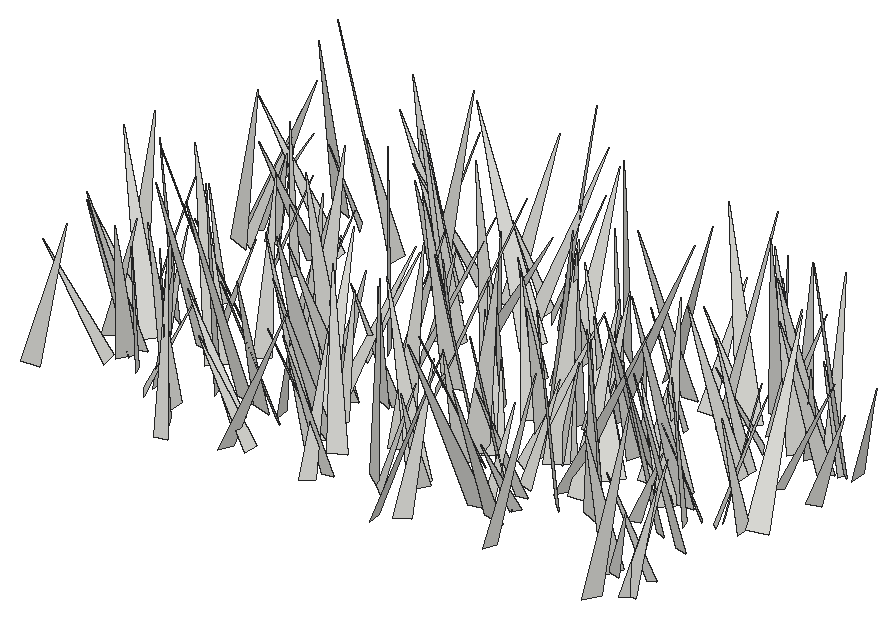
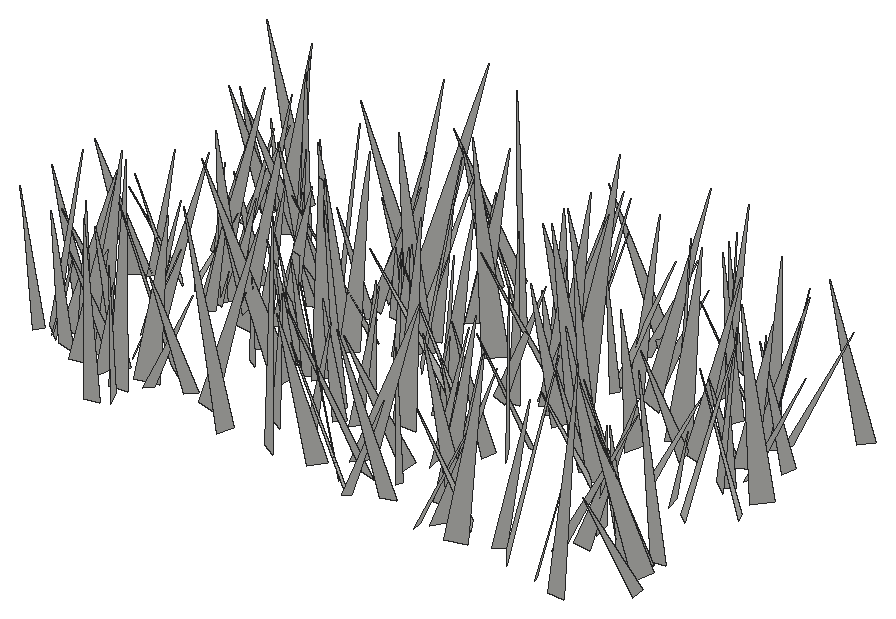
# SketchUp Ruby script. Lengths in inches.
U = 1.inch
M = Sketchup.active_model
def pt(a) = Geom::Point3d.new(a.map { |v| v * U })
def face(e, loops, mat)
  f = e.add_face(loops[0].map { |a| pt(a) })
  loops[1..].each { |l| e.add_face(l.map { |a| pt(a) }).erase! }
  f.material = f.back_material = mat if mat
  f
end
# faces: each face lists its corners as indices into pts; further lists are holes
def faces(e, pts, list, mat = nil) = list.each { |f| face(e, (f[0].is_a?(Array) ? f : [f]).map { |l| l.map { |i| pts[i] } }, mat) }
# xy, xz, yz: faces in a plane at the given z, y or x. An outline is a flat list of corners, or four numbers for a rectangle; further outlines are holes
def ring(l) = l.size == 4 ? [[l[0], l[1]], [l[2], l[1]], [l[2], l[3]], [l[0], l[3]]] : l.each_slice(2).to_a
def flat(e, list, mat, &to3) = list.each { |f| face(e, (f[0].is_a?(Array) ? f : [f]).map { |l| ring(l).map { |u, v| to3.(u, v) } }, mat) }
def xy(e, z, list, mat = nil) = flat(e, list, mat) { |x, y| [x, y, z] }
def xz(e, y, list, mat = nil) = flat(e, list, mat) { |x, z| [x, y, z] }
def yz(e, x, list, mat = nil) = flat(e, list, mat) { |y, z| [x, y, z] }
def lines(e, pts, list) = list.each { |a, b| e.add_line(pt(pts[a]), pt(pts[b])) }
# prism: a flat outline (further loops are holes) pulled along v
def prism(e, loops, v, mat = nil)
  f = face(e, loops, mat); d = Geom::Vector3d.new(v.map { |x| x * U })
  f.pushpull(f.normal.samedirection?(d) ? d.length : -d.length)
end
def box(e, o, s, mat = nil) = prism(e, [[o, [o[0] + s[0], o[1], o[2]], [o[0] + s[0], o[1] + s[1], o[2]], [o[0], o[1] + s[1], o[2]]]], [0, 0, s[2]], mat)
def at(x, y, z, deg = 0) = Geom::Transformation.translation(pt([x, y, z])) * Geom::Transformation.rotation(ORIGIN, Z_AXIS, deg.degrees)
def axes(o, x, y, z) = Geom::Transformation.new([*x, 0, *y, 0, *z, 0, *pt(o).to_a, 1])
def part(name) = M.definitions.add(name)
# library, detail: a bought-in or finely detailed component or shape, given as its bounding box
def library(name, o, s) = part(name).tap { |d| box(d.entities, o, s) }
def detail(e, o, s) = box(e.add_group.entities, o, s)
def put(e, d, t, mat = nil) = e.add_instance(d, t).tap { |i| i.material = mat if mat }
def group(e, t, mat = nil) = e.add_group.tap { |g| g.transformation = t; g.material = mat if mat }.entities
root = M.entities
c1 = part("fur_instance\#9")
p = [[0.8125,0,1.79],[0.67,-0.02,1.48],[0,-0.11,0],[0,0.11,0]]
faces(c1.entities,p,[[0,1,2,3]])
put(root,c1,axes([510.49,407.03,-21.66],[0.64289,6.12986,1.03372],[6.0316,-0.86662,1.38779],[-1.50455,-0.85491,6.00521]))
put(root,c1,axes([545.08,408,-21.66],[6.61649,-1.70465,2.3436],[-2.13195,-6.81989,1.0584],[-1.96294,1.66119,6.75008]))
put(root,c1,axes([515.89,409.48,-21.66],[-4.18794,0.93567,0.33129],[0.9893,4.05153,1.06324],[0.08071,-1.11073,4.15738]))
put(root,c1,axes([514.51,408.66,-21.66],[6.16079,-1.33707,0.34037],[-1.37023,-6.11166,0.79308],[-0.16154,0.84778,6.25413]))
put(root,c1,axes([527.73,407.37,-21.66],[6.18202,1.83786,0.77531],[1.68935,-6.16651,1.14736],[-1.06062,0.8903,6.34654]))
put(root,c1,axes([521.85,409.94,-21.66],[-1.08629,-5.09453,1.21583],[-5.17343,0.84989,-1.06105],[-0.81738,1.39139,5.09985]))
put(root,c1,axes([533.82,412.02,-21.66],[-0.13701,-6.93499,0.01519],[-6.899,0.13785,0.70555],[0.70571,0.00117,6.90036]))
put(root,c1,axes([509.59,409.04,-21.66],[4.32475,3.25099,2.86901],[3.37923,-5.06616,0.64681],[-2.71679,-1.12634,5.37159]))
put(root,c1,axes([532.06,412.72,-21.66],[1.01288,-8.11783,0.06805],[-8.08119,-1.01477,-0.77093],[-0.77341,-0.02823,8.14437]))
put(root,c1,axes([497.83,409.4,-21.66],[-1.7832,4.7887,2.83203],[5.02838,2.65983,-1.33139],[2.38064,-2.03113,4.93345]))
put(root,c1,axes([529.11,408.52,-21.66],[4.10356,-2.98524,2.70877],[-3.77942,-4.1935,1.10399],[-1.40181,2.56732,4.95298]))
put(root,c1,axes([544.13,411.4,-21.66],[4.71186,-4.25626,1.34995],[-4.06485,-4.9009,-1.26409],[-1.848,-0.07223,6.22249]))
put(root,c1,axes([546.75,409.71,-21.66],[-0.57371,3.97778,1.97621],[4.19128,1.14438,-1.08668],[1.47014,-1.71025,3.86924]))
put(root,c1,axes([508.65,410.58,-21.66],[-6.63003,0.58928,2.6026],[0.94805,7.03587,0.82207],[2.49439,-1.10786,6.6052]))
put(root,c1,axes([521.1875,408.62,-21.66],[-4.05743,3.11883,1.27429],[2.94276,4.25195,-1.03673],[1.64046,0.08657,5.0115]))
put(root,c1,axes([544.29,411.24,-21.66],[0.84418,-3.62493,0.18375],[-3.45271,-0.74384,1.18829],[1.11924,0.43944,3.52714]))
put(root,c1,axes([535.8,409.09,-21.66],[6.16496,0.12051,1.82007],[-0.27856,-6.27765,1.3592],[-1.80266,1.38221,6.01447]))
put(root,c1,axes([524.73,411.1,-21.66],[4.42565,6.01002,3.52258],[6.87552,-4.43985,-1.06317],[-1.12079,-3.50468,7.38759]))
put(root,c1,axes([525.68,410.375,-21.66],[2.6257,3.60497,0.95618],[3.72031,-2.44904,-0.98281],[0.26337,-1.34567,4.35019]))
put(root,c1,axes([546.72,409.49,-21.66],[4.55494,-1.38322,1.77977],[-1.90749,-4.50337,1.38185],[-1.20098,1.9065,4.55536]))
put(root,c1,axes([527.64,412.5,-21.66],[2.72704,-3.27265,0.76108],[-3.17295,-2.83078,-0.80329],[-1.10537,0.05182,4.1835]))
put(root,c1,axes([546.74,412.03,-21.66],[-0.5806,-4.0301,0.94816],[-3.96701,0.26756,-1.29192],[-1.18471,1.07913,3.86131]))
put(root,c1,axes([506.03,412.49,-21.66],[5.48101,-1.25937,0.85366],[-1.15676,-5.52263,-0.72019],[-0.98826,-0.52035,5.57753]))
put(root,c1,axes([505.86,411.0625,-21.66],[3.45283,2.51437,0.03768],[2.48973,-3.40925,-0.65094],[0.3531,-0.54815,4.22141]))
put(root,c1,axes([501.48,412.95,-21.66],[-4.90231,-0.23018,0.15933],[-0.18525,4.76264,1.18065],[0.20988,-1.17272,4.76358]))
put(root,c1,axes([512.93,411.9,-21.66],[-4.21656,2.08304,0.19454],[2.06998,4.09043,1.06765],[-0.30342,-1.04195,4.58024]))
put(root,c1,axes([518.06,413.75,-21.66],[-3.59271,-3.52154,0.36411],[-3.38524,3.56898,1.11534],[1.03633,-0.55007,4.90559]))
put(root,c1,axes([513.2,413.91,-21.66],[-0.67207,-6.04885,0.74296],[-6.03248,0.76649,0.78356],[0.86591,0.6451,6.03542]))
put(root,c1,axes([519.13,413.44,-21.66],[-0.74587,-6.40704,1.23448],[-6.45249,0.53969,-1.09751],[-0.96927,1.33753,6.35625]))
put(root,c1,axes([534.17,413.82,-21.66],[1.81992,-3.21241,0.00061],[-3.09433,-1.75321,-0.99152],[-0.86298,-0.48823,3.55649]))
put(root,c1,axes([502.11,413.96,-21.66],[4.76035,-4.27512,0.72339],[-4.20428,-4.81383,-0.78223],[-1.06017,-0.10597,6.35025]))
put(root,c1,axes([519.03,411.9,-21.66],[-7.32876,-0.97242,0.83606],[-1.07916,7.29688,-0.97277],[0.69283,1.07947,7.32872]))
put(root,c1,axes([511.65,414.28,-21.66],[-2.25691,-7.5793,1.44794],[-7.71352,2.17504,-0.63772],[-0.20948,1.56823,7.88243]))
put(root,c1,axes([515.05,413.35,-21.66],[-3.55918,-3.90599,0.48478],[-3.91702,3.45103,-0.95229],[-0.38568,0.99656,5.19785]))
put(root,c1,axes([527.17,412.74,-21.66],[-5.93712,3.87569,1.72238],[4.1151,5.9813,0.72589],[1.02637,-1.56207,7.0529]))
put(root,c1,axes([514.61,414.29,-21.66],[4.05285,-0.43746,0.41546],[-0.3233,-3.95717,-1.01285],[-0.50937,-0.96903,3.94856]))
put(root,c1,axes([501.86,414.7,-21.66],[-5.14482,-3.13912,1.24988],[-3.04737,5.29445,0.7535],[1.4594,-0.01101,5.97959]))
put(root,c1,axes([503.72,413.06,-21.66],[-3.72029,-1.54775,1.40082],[-1.82397,3.80239,-0.64288],[1.01535,1.15959,3.97778]))
put(root,c1,axes([520.62,412.48,-21.66],[-2.14866,5.91991,1.32548],[6.06222,2.04254,0.70466],[-0.22751,-1.48381,6.25824]))
put(root,c1,axes([533.73,413.79,-21.66],[-3.99562,-4.42007,1.47298],[-4.65768,3.83659,-1.12173],[0.11293,1.84803,5.85182]))
put(root,c1,axes([532.43,413.08,-21.66],[-0.05946,3.80591,1.08242],[3.88392,0.26301,-0.71143],[0.75616,-1.05166,3.7393]))
put(root,c1,axes([515.28,417.04,-21.66],[4.78768,-6.87101,0.53821],[-6.76798,-4.81092,-1.21319],[-1.30189,-0.25808,8.28619]))
put(root,c1,axes([502.28,415.18,-21.66],[-0.64276,-5.9949,1.38637],[-6.03632,0.34404,-1.31091],[-1.1932,1.48889,5.88502]))
put(root,c1,axes([533.38,415.46,-21.66],[-0.33962,-4.53633,0.58104],[-4.49375,0.22275,-0.88758],[-0.84975,0.63509,4.46159]))
put(root,c1,axes([509.49,414.14,-21.66],[-6.31517,-2.67121,2.41272],[-3.08957,6.52254,-0.86542],[1.84694,1.77736,6.80204]))
put(root,c1,axes([528.45,417.49,-21.66],[-3.25593,-5.45811,0.05054],[-5.36708,3.21208,1.12765],[0.99394,-0.53501,6.25464]))
put(root,c1,axes([539.3,416.14,-21.66],[-3.95013,-6.45103,2.53754],[-6.55598,4.42551,1.04517],[2.25256,1.56763,7.49179]))
put(root,c1,axes([538.61,416.06,-21.66],[-1.6159,-6.90986,2.38073],[-7.13771,2.01606,1.00679],[1.57067,2.05292,7.0245]))
put(root,c1,axes([527.76,416.44,-21.66],[3.7662,-3.06911,1.25827],[-2.92554,-3.97067,-0.92842],[-1.56328,0.03677,4.76883]))
put(root,c1,axes([523.4,415.52,-21.66],[-3.8242,6.03816,3.67075],[6.53219,4.61268,-0.78232],[2.69524,-2.61192,7.10435]))
put(root,c1,axes([499.39,415.42,-21.66],[4.23339,-1.74729,1.15695],[-1.93705,-4.25778,0.65751],[-0.79963,1.0637,4.53236]))
put(root,c1,axes([518.63,413.24,-21.66],[-3.78371,6.02543,0.57396],[5.96039,3.82698,-0.88298],[1.05307,-0.01122,7.05993]))
put(root,c1,axes([545.73,416.33,-21.66],[-2.90009,-5.61636,1.60668],[-5.82709,2.65472,-1.23809],[-0.41218,1.98605,6.19848]))
put(root,c1,axes([535.98,415.83,-21.66],[3.85266,4.81198,3.39076],[5.17881,-4.69725,0.78179],[-2.79863,-2.06788,6.11449]))
put(root,c1,axes([516.89,418.2,-21.66],[1.34944,-6.66989,1.0863],[-6.57389,-1.5523,-1.36482],[-1.56569,0.76902,6.66676]))
put(root,c1,axes([505.28,417.94,-21.66],[-1.29627,-6.42722,1.30707],[-6.54569,1.18361,-0.67151],[-0.41416,1.4099,6.52216]))
put(root,c1,axes([516.8,418.46,-21.66],[3.0521,-3.8403,0.46149],[-3.78154,-3.08617,-0.67208],[-0.8129,-0.06212,4.85917]))
put(root,c1,axes([541.03,417.4,-21.66],[2.68666,-2.71893,0.01615],[-2.65256,-2.616,0.85524],[0.59729,0.61233,3.72549]))
put(root,c1,axes([543.38,417.14,-21.66],[-3.32572,-4.76152,1.64129],[-5.0351,3.09772,-1.21581],[-0.11678,2.03921,5.67929]))
put(root,c1,axes([531.47,415.63,-21.66],[-0.67642,4.08917,0.12939],[3.98053,0.62749,0.97839],[-0.94522,-0.2838,4.0276]))
put(root,c1,axes([507.39,416.8,-21.66],[3.71191,-5.65782,4.04126],[-6.28277,-4.69165,-0.79764],[-2.97818,2.84578,6.7196]))
put(root,c1,axes([518.24,415.92,-21.66],[-3.95695,1.67084,0.9926],[1.45221,4.03835,-1.00857],[1.29152,0.5783,4.17516]))
put(root,c1,axes([532.73,416.59,-21.66],[0.16923,4.07191,1.2027],[4.12697,0.12503,-1.00402],[0.99752,-1.2081,3.94982]))
put(root,c1,axes([500.75,417.83,-21.66],[-4.62797,0.36048,0.06702],[0.36662,4.56134,0.78248],[0.00509,-0.78533,4.57556]))
put(root,c1,axes([527.45,418.07,-21.66],[5.01911,-5.50348,2.14134],[-5.83765,-5.04831,0.7082],[-0.89193,2.07156,7.41473]))
put(root,c1,axes([518.71,419.47,-21.66],[-0.89521,-5.51634,1.09126],[-5.41102,1.14576,1.35291],[1.53027,0.82431,5.42227]))
put(root,c1,axes([501.875,416.82,-21.66],[-4.84886,5.21937,0.60309],[5.25064,4.78392,0.8135],[-0.19034,-0.99462,7.07753]))
put(root,c1,axes([503.04,416.6875,-21.66],[-3.70619,1.07071,1.22273],[0.63141,3.75399,-1.37341],[1.4976,1.06701,3.605]))
put(root,c1,axes([526.24,419.6,-21.66],[-5.36571,-5.00333,1.81378],[-4.95811,5.63559,0.87824],[1.93398,0.5664,7.28374]))
put(root,c1,axes([535.12,417.54,-21.66],[7.55011,-1.58138,0.22082],[-1.59514,-7.42262,1.38345],[0.0711,1.39915,7.58887]))
put(root,c1,axes([515.36,418.99,-21.66],[3.59874,-6.83955,3.08177],[-7.12327,-4.18751,-0.97538],[-2.35281,2.21652,7.66674]))
put(root,c1,axes([501.02,419.45,-21.66],[0.91273,-4.1627,0.50654],[-4.12867,-0.80133,0.85424],[0.734,0.66898,4.1751]))
put(root,c1,axes([516.92,416.88,-21.66],[2.4518,5.85296,0.01413],[5.81055,-2.43218,-0.76857],[0.70347,-0.30989,6.29903]))
put(root,c1,axes([531.23,420.77,-21.66],[5.68928,-3.36377,1.44998],[-3.11585,-5.85243,-1.35122],[-1.92583,-0.46842,6.46971]))
put(root,c1,axes([519.79,419.6875,-21.66],[-0.88602,-4.48963,1.06047],[-4.46813,0.56653,-1.33464],[-1.14769,1.26043,4.37728]))
put(root,c1,axes([505.84,418.125,-21.66],[4.17653,-0.25853,0.87813],[-0.4857,-4.1025,1.10224],[-0.77592,1.17643,4.03674]))
put(root,c1,axes([536.4,417.51,-21.66],[-1.26821,6.79621,1.34265],[6.86908,1.41065,-0.65215],[0.89826,-1.19212,6.8827]))
put(root,c1,axes([528.29,418.43,-21.66],[-1.05429,4.67357,0.99792],[4.75005,0.91265,0.74413],[-0.52453,-1.12891,4.73287]))
put(root,c1,axes([543.76,419.17,-21.66],[-4.56501,-1.69942,1.47091],[-1.97129,4.62695,-0.77219],[1.07964,1.26263,4.80947]))
put(root,c1,axes([514.65,419.9,-21.66],[3.82808,-2.96393,0.87418],[-3.08142,-3.76593,0.72521],[-0.23226,1.11183,4.78677]))
put(root,c1,axes([538.39,422.63,-21.66],[-2.04467,-7.63412,0.65301],[-7.56547,2.11851,1.07815],[1.21235,0.345,7.82931]))
put(root,c1,axes([542.29,420.97,-21.66],[-1.50167,-7.67594,2.08534],[-7.92089,1.24921,-1.10571],[-0.72669,2.24569,7.7429]))
put(root,c1,axes([501.56,419.78,-21.66],[-3.6941,-4.73944,2.34113],[-5.23892,3.66336,-0.85037],[0.70493,2.38895,5.94858]))
put(root,c1,axes([498.17,419.72,-21.66],[4.86014,-4.74094,2.82615],[-5.30574,-5.05065,0.65171],[-1.52079,2.46963,6.75816]))
put(root,c1,axes([547.31,420.81,-21.66],[-4.17455,0.44699,1.70239],[0.80041,4.38471,0.81146],[1.56757,-1.04848,4.11925]))
put(root,c1,axes([544.33,420.21,-21.66],[-3.00148,-2.27694,0.1564],[-2.20162,2.82047,-1.1898],[-0.60148,1.03841,3.57459]))
put(root,c1,axes([532.32,420.63,-21.66],[2.08402,3.38406,1.47593],[3.68931,-1.84524,-0.97848],[0.13865,-1.76538,3.85196]))
put(root,c1,axes([541.26,420.34,-21.66],[-2.68831,3.38264,1.06218],[3.54497,2.54168,0.8778],[-0.06058,-1.37662,4.23069]))
put(root,c1,axes([530.9,418.625,-21.66],[2.76171,5.55128,0.00194],[5.48471,-2.72826,-0.95829],[0.85713,-0.42855,6.1258]))
put(root,c1,axes([528.06,419.45,-21.66],[-1.29816,5.29172,0.79515],[5.27739,1.13069,1.0911],[-0.88529,-1.01932,5.33826]))
put(root,c1,axes([508.99,419.29,-21.66],[-5.25856,3.05312,1.43062],[2.8843,5.44607,-1.02073],[1.74617,0.1987,5.99435]))
put(root,c1,axes([510.94,421.44,-21.66],[0.6303,-6.24139,2.24897],[-6.57772,-0.29373,1.02832],[0.86396,2.31708,6.18828]))
put(root,c1,axes([512.25,420.5,-21.66],[-3.47776,6.78239,3.15196],[7.08859,4.09761,-0.99596],[2.38486,-2.28893,7.55669]))
put(root,c1,axes([532.37,420.26,-21.66],[-5.26533,5.42334,2.66225],[5.51698,5.75546,-0.81326],[2.46233,-1.29842,7.51498]))
put(root,c1,axes([505.51,421.85,-21.66],[-2.7303,-2.91554,0.15676],[-2.8364,2.59761,-1.08937],[-0.69267,0.85529,3.84294]))
put(root,c1,axes([541.29,420.16,-21.66],[-5.91196,3.62871,1.99788],[3.48429,6.23911,-1.02156],[2.24027,-0.12769,6.86114]))
put(root,c1,axes([541.53,422.24,-21.66],[-3.71371,1.13934,1.58672],[1.47505,3.87017,0.67337],[1.28063,-1.15373,3.82574]))
put(root,c1,axes([498.09,422.06,-21.66],[4.56554,2.4835,0.72557],[2.58092,-4.47494,-0.92307],[-0.18188,-1.15993,5.11467]))
put(root,c1,axes([545.45,420.15,-21.66],[3.29969,3.36632,0.10349],[3.25213,-3.22241,1.12716],[-0.87548,0.71745,4.57707]))
put(root,c1,axes([532.77,421.125,-21.66],[1.28068,6.67783,2.12971],[6.86225,-1.63556,1.00185],[-1.42781,-1.87102,6.72532]))
put(root,c1,axes([536.59,420.875,-21.66],[-4.59485,5.55244,0.46156],[5.5505,4.50971,1.00485],[-0.48434,-0.99407,7.1367]))
put(root,c1,axes([535.84,424.08,-21.66],[4.30794,-3.29071,0.86204],[-3.07513,-4.36194,-1.28347],[-1.45447,-0.52435,5.26686]))
put(root,c1,axes([545.42,421.13,-21.66],[3.89268,2.82638,0.90518],[2.67493,-3.98806,0.94914],[-1.28551,0.26015,4.71599]))
put(root,c1,axes([500.9,424.45,-21.66],[-3.86726,-4.8383,0.71579],[-4.78645,3.93151,0.71436],[1.00566,0.10641,6.1526]))
put(root,c1,axes([534.05,423.86,-21.66],[4.56733,-2.95407,1.62637],[-2.80415,-4.84794,-0.93072],[-1.87305,0.05455,5.35918]))
put(root,c1,axes([525.3,423.53,-21.66],[-4.30625,-1.78107,2.16646],[-1.55574,4.81995,0.87021],[2.33354,-0.07334,4.57807]))
put(root,c1,axes([538.29,421.9,-21.66],[-1.13275,3.97734,1.11963],[3.98013,1.3621,-0.81189],[1.10966,-0.82546,4.05502]))
put(root,c1,axes([521.09,423.81,-21.66],[0.92373,-7.0899,2.33425],[-7.39568,-1.18748,-0.68009],[-1.00963,2.21177,7.11741]))
put(root,c1,axes([530.23,424.52,-21.66],[7.09602,-3.54407,1.49132],[-3.45875,-7.25092,-0.77408],[-1.67974,-0.04148,7.89397]))
put(root,c1,axes([520.56,424.66,-21.66],[-2.364,-4.99525,1.36106],[-4.8414,2.66304,1.36474],[1.83462,0.59091,5.35523]))
put(root,c1,axes([532.5,423.86,-21.66],[4.32257,0.5968,0.21737],[0.63053,-4.21214,-0.97382],[-0.07654,-0.99484,4.25352]))
put(root,c1,axes([508.21,424.18,-21.66],[4.08731,-3.32744,0.79787],[-3.41978,-4.01464,0.77613],[-0.11643,1.10699,5.21302]))
put(root,c1,axes([509.62,423.59,-21.66],[-0.91828,3.53646,1.4047],[3.57282,1.29857,-0.93362],[1.30946,-1.06309,3.53244]))
put(root,c1,axes([531.29,424.83,-21.66],[1.4619,-3.63585,0.57448],[-3.60479,-1.28901,1.01518],[0.74496,0.89757,3.78497]))
put(root,c1,axes([548.03,421.25,-21.66],[-3.4412,6.39637,0.09759],[6.32165,3.41718,-1.06042],[0.97968,0.41743,7.18546]))
put(root,c1,axes([502.64,423.27,-21.66],[-3.94683,-0.00707,0.27926],[-0.08275,3.80753,-1.07302],[0.26682,1.07619,3.79817]))
put(root,c1,axes([514.09,423.42,-21.66],[2.1149,3.97719,0.39309],[3.90996,-1.96694,-1.13523],[0.82754,-0.87089,4.35914]))
put(root,c1,axes([527.41,423.57,-21.66],[-1.32199,4.73147,0.88748],[4.77716,1.17578,0.84759],[-0.59431,-1.0737,4.83901]))
put(root,c1,axes([542.96,425.77,-21.66],[-6.41083,1.14128,1.69671],[1.48537,6.43646,1.28286],[1.40536,-1.59673,6.38401]))
put(root,c1,axes([520.5,422.61,-21.66],[5.97415,4.42308,0.10738],[4.35531,-5.91092,1.16532],[-0.77872,0.87356,7.3414]))
put(root,c1,axes([532.86,424.31,-21.66],[3.50267,-1.34823,2.1537],[-1.97697,-3.75014,0.86764],[-1.59615,1.68627,3.65152]))
put(root,c1,axes([532.64,424.18,-21.66],[-1.16488,5.07104,1.08343],[5.11451,1.30667,-0.61696],[0.85504,-0.90739,5.16641]))
put(root,c1,axes([548.65,426.32,-21.66],[3.25053,-3.28963,0.28157],[-3.26975,-3.15258,0.91484],[0.45796,0.84053,4.53329]))
put(root,c1,axes([517.09,425.46,-21.66],[5.75926,3.61485,0.22209],[3.58079,-5.62103,-1.36658],[0.54262,-1.27375,6.66098]))
put(root,c1,axes([514.87,424.99,-21.66],[-5.7993,-3.05465,2.69516],[-3.68736,5.92923,-1.21419],[1.7315,2.39584,6.44116]))
put(root,c1,axes([508.36,424.47,-21.66],[3.43862,2.40363,0.16823],[2.31203,-3.37399,0.94893],[-0.67841,0.6845,4.08669]))
put(root,c1,axes([515.74,425.78,-21.66],[4.66394,-1.20705,1.00362],[-1.36601,-4.67089,0.73033],[-0.77347,0.97077,4.76192]))
put(root,c1,axes([522.29,426.28,-21.66],[0.36283,-7.33481,3.26148],[-7.98321,-0.67122,-0.62142],[-0.83968,3.21222,7.31744]))
put(root,c1,axes([526.73,427.16,-21.66],[6.91292,1.02767,1.79019],[1.3308,-7.00178,-1.11957],[-1.57792,-1.40299,6.89863]))
put(root,c1,axes([542.87,426.91,-21.66],[-4.85785,0.78834,1.37895],[1.02249,4.94749,0.77364],[1.21552,-1.0112,4.86021]))
put(root,c1,axes([535.15,425.81,-21.66],[1.49909,3.09185,1.25062],[3.12666,-1.78006,0.6529],[-1.16087,-0.8017,3.3735]))
put(root,c1,axes([503.24,426.81,-21.66],[4.3525,2.53578,0.43229],[2.57081,-4.2585,-0.90411],[0.08934,-0.99816,4.9555]))
put(root,c1,axes([531.91,426.54,-21.66],[7.97011,-1.5942,0.50435],[-1.65185,-7.88792,1.1707],[-0.25934,1.24806,8.04323]))
put(root,c1,axes([524.85,428.03,-21.66],[4.20178,-1.75309,2.00996],[-1.5081,-4.65512,-0.90755],[-2.19975,-0.15714,4.46146]))
put(root,c1,axes([545.625,426.61,-21.66],[4.34496,-0.35551,0.43941],[-0.4633,-4.19131,1.19014],[-0.32376,1.22666,4.19388]))
put(root,c1,axes([526.01,428.25,-21.66],[2.52401,-3.24586,0.70539],[-3.32076,-2.44552,0.62916],[0.07602,0.94215,4.0633]))
put(root,c1,axes([516.17,427.91,-21.66],[2.59266,-2.6088,0.97622],[-2.78019,-2.50569,0.68761],[-0.17141,1.18171,3.61316]))
put(root,c1,axes([541.58,429.99,-21.66],[-3.32799,-2.15223,0.18164],[-2.02775,3.22824,1.09879],[0.74386,-0.82886,3.80792]))
put(root,c1,axes([546.8,429.85,-21.66],[0.96308,-5.75121,1.64983],[-5.7805,-1.32563,-1.24675],[-1.54408,1.37555,5.69645]))
put(root,c1,axes([536.19,428.78,-21.66],[-3.92472,-1.58946,0.29836],[-1.61245,3.78584,-1.04222],[-0.12416,1.07696,4.10409]))
put(root,c1,axes([517.86,428.54,-21.66],[-6.43885,-0.2283,0.73687],[-0.34147,6.39798,-1.00159],[0.69173,1.03328,6.36457]))
put(root,c1,axes([498.43,430,-21.66],[1.5633,5.69815,3.01797],[6.40687,-1.02237,-1.38843],[0.72737,-3.24142,5.74326]))
put(root,c1,axes([544.76,430.96,-21.66],[3.91329,-2.80057,0.16354],[-2.76188,-3.89534,-0.61821],[-0.49189,-0.40864,4.7723]))
put(root,c1,axes([503.64,431.38,-21.66],[0.77993,-5.26102,0.56712],[-5.12867,-0.89269,-1.22806],[-1.30258,0.36472,5.1748]))
put(root,c1,axes([548.64,430.84,-21.66],[4.67229,-0.63233,0.28263],[-0.57173,-4.60903,-0.86025],[-0.39095,-0.81674,4.63574]))
put(root,c1,axes([503.98,428.92,-21.66],[-5.02502,0.15502,0.9974],[-0.08895,4.97687,-1.22169],[1.00545,1.21508,4.87671]))
put(root,c1,axes([500.14,431.37,-21.66],[2.04033,-4.0488,0.48109],[-4.03745,-1.93127,0.8697],[0.56854,0.81522,4.44965]))
put(root,c1,axes([525.71,431.81,-21.66],[-3.46561,0.71078,2.1355],[1.4755,3.67824,1.17025],[1.69955,-1.74395,3.33859]))
put(root,c1,axes([543.7,431.02,-21.66],[-5.4764,4.5647,2.90915],[5.14181,5.68019,0.76664],[1.69155,-2.48788,7.08799]))
put(root,c1,axes([518.8,430.14,-21.66],[4.72114,-1.50275,0.05764],[-1.46013,-4.53503,1.361],[0.36002,1.31378,4.76394]))
put(root,c1,axes([547.63,430.64,-21.66],[-4.59653,-5.39297,2.39685],[-5.86856,4.49796,-1.13384],[0.62378,2.57709,6.99476]))
put(root,c1,axes([533.8,432.18,-21.66],[-0.89834,-6.55906,1.37521],[-6.65422,0.70817,-0.96916],[-0.7961,1.48213,6.54897]))
put(root,c1,axes([547.69,430.35,-21.66],[-3.7674,-0.4134,0.34529],[-0.49063,3.64055,-0.99453],[0.22227,1.02903,3.6572]))
put(root,c1,axes([501.4,430.33,-21.66],[-2.88957,-1.62735,2.00469],[-2.2228,3.09866,-0.68855],[1.31385,1.66334,3.24403]))
put(root,c1,axes([543.88,432.57,-21.66],[2.81422,-5.9892,1.8303],[-5.99838,-3.15452,-1.09945],[-1.79999,1.14839,6.52546]))
put(root,c1,axes([517.93,432.24,-21.66],[4.34491,0.59069,1.09524],[0.90101,-4.23706,-1.28924],[-0.85828,-1.45776,4.19106]))
put(root,c1,axes([512.7,433.07,-21.66],[2.86729,-4.50295,0.62999],[-4.43501,-2.93396,-0.78577],[-1.00209,0.10064,5.2802]))
put(root,c1,axes([498.9,430.34,-21.66],[2.45412,4.72767,0.6627],[4.74881,-2.3413,-0.8831],[0.48874,-0.99004,5.25297]))
put(root,c1,axes([513.9375,432.61,-21.66],[1.75802,-6.33898,1.96931],[-6.51413,-2.03906,-0.74828],[-1.27556,1.67662,6.53555]))
put(root,c1,axes([529.01,431.06,-21.66],[1.89742,4.59885,2.05217],[4.78177,-2.33318,0.8074],[-1.57969,-1.53878,4.90894]))
put(root,c1,axes([504.62,432.51,-21.66],[-6.1435,0.43905,0.01492],[0.43419,6.03663,1.1429],[-0.06685,-1.14104,6.05221]))
put(root,c1,axes([541.01,431.73,-21.66],[4.40781,-2.35415,1.32075],[-2.57038,-4.43283,0.67704],[-0.82436,1.23418,4.95101]))
put(root,c1,axes([538.34,432.42,-21.66],[-3.99734,1.08155,0.32432],[1.12476,3.91891,0.79421],[0.09918,-0.85212,4.0642]))
put(root,c1,axes([498.08,432,-21.66],[6.2285,-2.9564,0.62521],[-3.02175,-6.08711,1.31964],[0.01382,1.46019,6.76705]))
put(root,c1,axes([538.09,429.875,-21.66],[3.95249,6.61953,0.92655],[6.54498,-4.05132,1.02412],[-1.35642,-0.25967,7.64143]))
put(root,c1,axes([539.79,433.76,-21.66],[-0.40221,-7.56998,1.93164],[-7.73436,0.65878,0.97125],[1.10251,1.85984,7.51818]))
put(root,c1,axes([521.65,431.26,-21.66],[-7.18183,4.15456,0.03319],[4.14203,7.15453,0.70461],[-0.3242,-0.62648,8.26695]))
put(root,c1,axes([535.7,431.36,-21.66],[-1.59343,4.55905,1.08338],[4.45907,1.82697,-1.12985],[1.44061,-0.61229,4.69546]))
put(root,c1,axes([530.95,433.8,-21.66],[7.51831,-0.309,0.51299],[-0.23256,-7.46002,-1.08516],[-0.55186,-1.06592,7.446]))
put(root,c1,axes([527.25,433.99,-21.66],[-3.84702,-6.56229,2.86732],[-6.71624,4.43571,1.14075],[2.48541,1.82909,7.52076]))
put(root,c1,axes([538.89,431.9375,-21.66],[2.27452,-5.56414,4.58515],[-6.58849,-3.55674,-1.04785],[-2.92831,3.68058,5.91904]))
put(root,c1,axes([541.07,431.96,-21.66],[4.54007,-1.04122,1.07478],[-1.33062,-4.37982,1.37772],[-0.68465,1.60765,4.44952]))
put(root,c1,axes([545.71,431.66,-21.66],[0.35449,6.1752,1.09899],[6.2119,-0.49795,0.79425],[-0.86782,-1.04187,6.13416]))
put(root,c1,axes([507.69,434.74,-21.66],[-4.50462,1.14541,2.32905],[1.86637,4.67145,1.31236],[1.80364,-1.97324,4.45884]))
put(root,c1,axes([512.69,434.82,-21.66],[-6.22259,1.31552,1.1088],[1.51746,6.15727,1.21077],[0.81078,-1.42761,6.24382]))
put(root,c1,axes([541.85,432.83,-21.66],[-4.80614,1.67739,0.07303],[1.63862,4.73444,-0.90443],[0.36591,0.83033,5.00945]))
put(root,c1,axes([513.59,435.85,-21.66],[-4.70083,-1.74871,0.0814],[-1.70109,4.61801,0.97093],[0.41342,-0.88228,4.92068]))
put(root,c1,axes([512.04,433.26,-21.66],[6.62959,-1.41825,2.66639],[-1.99694,-6.88369,1.30369],[-2.26567,1.91728,6.65307]))
put(root,c1,axes([497.02,433.92,-21.66],[3.6219,-1.04912,0.12415],[-1.02885,-3.40219,1.26523],[0.23987,1.24847,3.55218]))
put(root,c1,axes([519.67,435.42,-21.66],[-3.46593,0.7925,0.89611],[1.04093,3.35143,1.06213],[0.58952,-1.25841,3.39303]))
put(root,c1,axes([520.2,432.64,-21.66],[2.81698,6.47491,0.35167],[6.46114,-2.77024,-0.75032],[0.54938,-0.62035,7.02117]))
put(root,c1,axes([523.62,433.5,-21.66],[-3.09006,5.24053,1.65653],[5.13422,3.43055,-1.27548],[1.9614,-0.72379,5.94851]))
put(root,c1,axes([506.57,435.43,-21.66],[-6.42891,-4.93695,1.78859],[-5.18873,6.40682,-0.96596],[0.80598,1.86616,8.04806]))
put(root,c1,axes([503.27,436.54,-21.66],[-3.15969,-2.10838,0.70871],[-1.88389,3.19122,1.09464],[1.18257,-0.54957,3.6374]))
put(root,c1,axes([540.09,436.04,-21.66],[0.10364,-5.95888,1.80759],[-6.13378,0.21397,1.05707],[1.07352,1.79787,5.86529]))
put(root,c1,axes([521.94,433.61,-21.66],[5.36611,5.59511,2.05394],[5.5109,-5.71038,1.15783],[-2.27022,-0.63666,7.66549]))
put(root,c1,axes([520.3,434.875,-21.66],[4.29759,3.17988,0.45483],[3.21134,-4.23507,-0.73441],[0.07624,-0.86047,5.29543]))
put(root,c1,axes([517.2,434.3,-21.66],[0.34617,6.42334,1.62872],[6.51894,-0.03728,-1.2385],[1.18972,-1.66468,6.31231]))
put(root,c1,axes([510.375,435.92,-21.66],[-3.35147,5.54659,2.9979],[6.27053,3.28643,0.92965],[0.65767,-3.06906,6.41348]))
put(root,c1,axes([500.9,437.48,-21.66],[-1.7083,-7.51191,1.45388],[-7.48357,1.95063,1.28533],[1.59333,1.10775,7.59572]))
put(root,c1,axes([510.85,433.61,-21.66],[4.46685,2.95329,0.59597],[2.75098,-4.43263,1.34675],[-1.2285,0.81223,5.18275]))
put(root,c1,axes([539.26,434.92,-21.66],[-4.67336,-1.61213,2.14084],[-2.03116,4.93814,-0.71533],[1.7483,1.42769,4.89159]))
